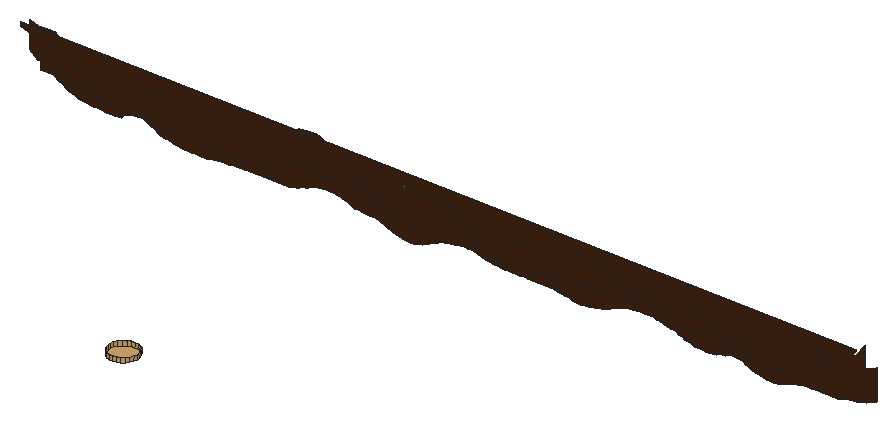
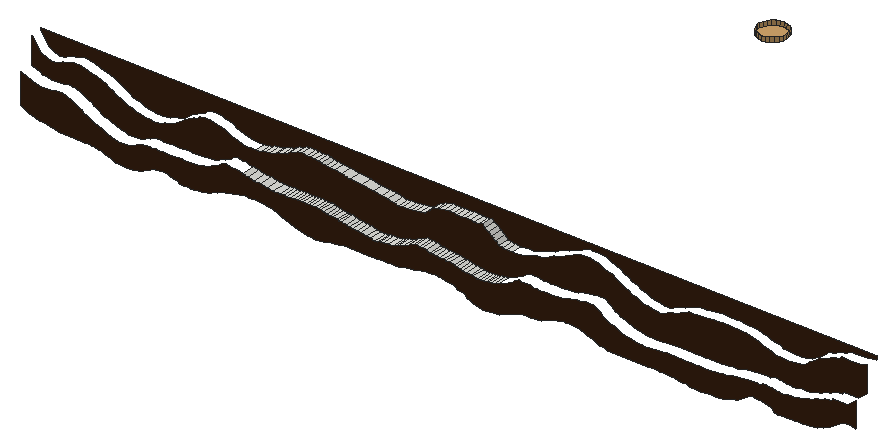
# SketchUp Ruby script. Lengths in inches.
U = 1.inch
M = Sketchup.active_model
def pt(a) = Geom::Point3d.new(a.map { |v| v * U })
def face(e, loops, mat)
  f = e.add_face(loops[0].map { |a| pt(a) })
  loops[1..].each { |l| e.add_face(l.map { |a| pt(a) }).erase! }
  f.material = f.back_material = mat if mat
  f
end
# faces: each face lists its corners as indices into pts; further lists are holes
def faces(e, pts, list, mat = nil) = list.each { |f| face(e, (f[0].is_a?(Array) ? f : [f]).map { |l| l.map { |i| pts[i] } }, mat) }
# xy, xz, yz: faces in a plane at the given z, y or x. An outline is a flat list of corners, or four numbers for a rectangle; further outlines are holes
def ring(l) = l.size == 4 ? [[l[0], l[1]], [l[2], l[1]], [l[2], l[3]], [l[0], l[3]]] : l.each_slice(2).to_a
def flat(e, list, mat, &to3) = list.each { |f| face(e, (f[0].is_a?(Array) ? f : [f]).map { |l| ring(l).map { |u, v| to3.(u, v) } }, mat) }
def xy(e, z, list, mat = nil) = flat(e, list, mat) { |x, y| [x, y, z] }
def xz(e, y, list, mat = nil) = flat(e, list, mat) { |x, z| [x, y, z] }
def yz(e, x, list, mat = nil) = flat(e, list, mat) { |y, z| [x, y, z] }
def lines(e, pts, list) = list.each { |a, b| e.add_line(pt(pts[a]), pt(pts[b])) }
# prism: a flat outline (further loops are holes) pulled along v
def prism(e, loops, v, mat = nil)
  f = face(e, loops, mat); d = Geom::Vector3d.new(v.map { |x| x * U })
  f.pushpull(f.normal.samedirection?(d) ? d.length : -d.length)
end
def box(e, o, s, mat = nil) = prism(e, [[o, [o[0] + s[0], o[1], o[2]], [o[0] + s[0], o[1] + s[1], o[2]], [o[0], o[1] + s[1], o[2]]]], [0, 0, s[2]], mat)
def at(x, y, z, deg = 0) = Geom::Transformation.translation(pt([x, y, z])) * Geom::Transformation.rotation(ORIGIN, Z_AXIS, deg.degrees)
def axes(o, x, y, z) = Geom::Transformation.new([*x, 0, *y, 0, *z, 0, *pt(o).to_a, 1])
def part(name) = M.definitions.add(name)
# library, detail: a bought-in or finely detailed component or shape, given as its bounding box
def library(name, o, s) = part(name).tap { |d| box(d.entities, o, s) }
def detail(e, o, s) = box(e.add_group.entities, o, s)
def put(e, d, t, mat = nil) = e.add_instance(d, t).tap { |i| i.material = mat if mat }
def group(e, t, mat = nil) = e.add_group.tap { |g| g.transformation = t; g.material = mat if mat }.entities
root = M.entities
M.materials.add("[Field Square Tile]").color = [211, 167, 108]
M.materials.add("[Wood Veneer 01]").color = [66, 38, 20]
xy(root,243.05,[[358.29,2398.8,358.97,2401.37]])
xy(root,243.07,[[356.4375,2398.8,357.02,2401.37]])
xy(root,243.09,[[353.125,2398.8,353.65,2401.37],[353.65,2398.8,354.17,2401.37],[354.17,2398.8,354.83,2401.37],[354.83,2398.8,355.28,2401.37]])
xy(root,249.21,[[325.92,2396.68,326.81,2398.8]])
xy(root,249.22,[[327.53,2396.68,328.4375,2398.8]])
xy(root,249.23,[[329.08,2396.68,329.98,2398.8]])
xy(root,250.6875,[[324.47,2328.39,323.81,2328.48,323.19,2328.74,322.66,2329.14,322.25,2329.68,322,2330.29,321.91,2330.96,322,2331.62,322.25,2332.24,322.66,2332.77,323.19,2333.18,323.81,2333.43,324.47,2333.52,325.13,2333.43,325.75,2333.18,326.28,2332.77,326.69,2332.24,326.95,2331.62,327.03,2330.96,326.95,2330.29,326.69,2329.68,326.28,2329.14,325.75,2328.74,325.13,2328.48]],"[Field Square Tile]")
xz(root,2396.68,[[384.34,244.87,385.25,245.01,386.1875,245.12,386.95,245.25,387.71,245.41,388.34,245.78,389.14,245.88,389.85,246.16,390.45,246.57,391.24,246.9,391.84,247.35,392.51,247.62,393.1,248.06,393.86,248.32,394.97,248.66,395.75,248.79,396.61,249.19,397.28,249.32,398.21,249.41,399.06,249.48,399.81,249.21,400.45,248.96,401.15,248.9,401.95,248.42,402.66,248.3,403.37,248.22,404.1875,248.56,405.12,249.02,406.85,251.16,406.85,251.5,252.84,251.5,252.84,250.88,254.43,250.53,256.05,250.54,257.51,250.55,258.04,250.15,258.65,249.97,259.45,249.8,260.12,249.41,260.79,249.2,261.56,249.01,262.05,248.51,262.68,248.07,263.33,247.72,263.97,247.25,264.52,246.88,265.24,246.73,265.9,246.62,266.64,246.54,267.42,246.51,268.2,246.58,269,246.59,269.8,246.69,270.51,247.03,271.2,247.2,272.17,247.39,272.8,247.78,273.58,247.89,274.58,248.18,275.22,248.29,276.11,248.35,276.84,248.4,277.83,248.4375,278.49,248.46,279.38,248.47,280.12,248.48,281.01,248.49,281.74,248.39,283.14,248.28,284.17,248.15,284.99,248.11,285.79,248.08,286.63,247.66,287.26,247.46,287.94,247.08,288.625,246.94,289.48,246.66,290.09,246.35,290.86,246.05,291.76,246.13,292.47,246.29,293.27,246.41,294.18,246.55,294.91,246.92,295.52,247.12,296.2,247.31,296.77,247.71,297.7,248.03,298.41,248.46,299.19,248.82,299.91,249.37,300.7,249.5625,301.6,249.9,302.52,250.35,303.18,250.49,303.99,250.6,305.01,250.58,305.65,250.61,306.27,250.32,306.96,250.0625,307.62,249.68,308.38,249.46,309.27,248.95,310.49,248.69,311.4,248.26,312,247.9,313.13,247.66,313.71,247.53,314.39,247.25,315.2,246.95,315.89,246.75,316.68,246.66,317.39,246.59,318.28,246.55,319.21,246.63,319.95,246.74,320.68,246.87,321.29,247.42,321.96,247.96,322.53,248.44,323.27,248.85,323.74,249.34,324.47,249.125,325.24,249.17,325.92,249.21,326.81,249.21,327.53,249.22,328.4375,249.22,329.08,249.23,329.98,249.23,330.72,249.24,331.52,249.14,332.15,248.82,332.94,248.54,333.64,248.04,334.33,247.48,335.22,247.29,336.04,247.15,336.77,247.05,337.49,247,338.4,246.96,339.125,246.94,340.04,247.04,341.1,247.36,342.28,247.43,343.93,247.6,345.91,247.98,348.11,248.1875,349.72,248.49,350.97,248.62,351.91,248.69,352.59,248.75,353.25,249.09,353.95,249.18,354.73,249.13,355.43,249.17,356.13,249.18,357.03,249.29,357.76,249.21,358.37,248.8,359.0625,248.73,359.84,248.26,360.54,248.02,361.34,247.8125,362.05,247.4,362.96,247.27,363.7,247.18,364.625,246.91,365.49,246.84,366.44,246.79,367.22,246.75,367.97,246.83,369.01,247.25,369.88,247.55,370.55,247.66,371.18,248.16,371.97,248.41,372.67,248.52,373.37,248.72,374.07,248.8,374.96,248.85,375.79,248.6875,376.33,248.26,377.02,248.06,377.91,247.55,378.62,247.19,379.43,246.63,380.0625,246.13,380.65,245.83,381.33,245.67,382.2,245.46,382.91,245.0625,383.625,244.95]],"[Wood Veneer 01]")
xz(root,2398.8,[[388.34,241.09,388.91,241.14,389.55,241.35,390.14,241.46,391.08,241.85,392.08,242.23,392.64,242.42,393.36,242.61,393.875,242.91,394.25,243.14,394.79,243.52,395.27,243.71,395.6,244.02,396.04,244.21,396.63,244.57,397.1,244.76,397.72,245.125,398.22,245.32,398.7,245.41,399.25,245.48,399.74,245.59,400.27,245.55,400.88,245.35,401.37,245.31,401.92,245.27,402.48,245.24,403.04,245.22,403.6,245.34,404.23,245.42,404.8125,245.52,405.19,245.76,405.66,245.9,406.85,246.43,406.85,251.16,405.12,249.02,404.1875,248.56,403.37,248.22,402.66,248.3,401.95,248.42,401.15,248.9,400.45,248.96,399.81,249.21,399.06,249.48,398.21,249.41,397.28,249.32,396.61,249.19,395.75,248.79,394.97,248.66,393.86,248.32,393.1,248.06,392.51,247.62,391.84,247.35,391.24,246.9,390.45,246.57,389.85,246.16,389.14,245.88,388.34,245.78,387.71,245.41,386.95,245.25,386.1875,245.12,385.25,245.01,384.34,244.87,383.625,244.95,382.91,245.0625,382.2,245.46,381.33,245.67,380.65,245.83,380.0625,246.13,379.43,246.63,378.62,247.19,377.91,247.55,377.02,248.06,376.33,248.26,375.79,248.6875,374.96,248.85,374.07,248.8,373.37,248.72,372.67,248.52,371.97,248.41,371.18,248.16,370.55,247.66,369.88,247.55,369.01,247.25,367.97,246.83,367.22,246.75,366.44,246.79,365.49,246.84,364.625,246.91,363.7,247.18,362.96,247.27,362.05,247.4,361.34,247.8125,360.54,248.02,359.84,248.26,359.0625,248.73,358.37,248.8,357.76,249.21,357.03,249.29,356.13,249.18,355.43,249.17,354.73,249.13,353.95,249.18,353.25,249.09,352.59,248.75,351.91,248.69,350.97,248.62,349.72,248.49,348.11,248.1875,345.91,247.98,343.93,247.6,342.28,247.43,341.1,247.36,340.04,247.04,339.125,246.94,338.4,246.96,337.49,247,336.77,247.05,336.04,247.15,335.22,247.29,334.33,247.48,333.64,248.04,332.94,248.54,332.15,248.82,331.52,249.14,330.72,249.24,329.98,249.23,329.08,249.23,328.4375,249.22,327.53,249.22,326.81,249.21,325.92,249.21,325.24,249.17,324.47,249.125,323.74,249.34,323.27,248.85,322.53,248.44,321.96,247.96,321.29,247.42,320.68,246.87,319.95,246.74,319.21,246.63,318.28,246.55,317.39,246.59,316.68,246.66,315.89,246.75,315.2,246.95,314.39,247.25,313.71,247.53,313.13,247.66,312,247.9,311.4,248.26,310.49,248.69,309.27,248.95,308.38,249.46,307.62,249.68,306.96,250.0625,306.27,250.32,305.65,250.61,305.01,250.58,303.99,250.6,303.18,250.49,302.52,250.35,301.6,249.9,300.7,249.5625,299.91,249.37,299.19,248.82,298.41,248.46,297.7,248.03,296.77,247.71,296.2,247.31,295.52,247.12,294.91,246.92,294.18,246.55,293.27,246.41,292.47,246.29,291.76,246.13,290.86,246.05,290.09,246.35,289.48,246.66,288.625,246.94,287.94,247.08,287.26,247.46,286.63,247.66,285.79,248.08,284.99,248.11,284.17,248.15,283.14,248.28,281.74,248.39,281.01,248.49,280.12,248.48,279.38,248.47,278.49,248.46,277.83,248.4375,276.84,248.4,276.11,248.35,275.22,248.29,274.58,248.18,273.58,247.89,272.8,247.78,272.17,247.39,271.2,247.2,270.51,247.03,269.8,246.69,269,246.59,268.2,246.58,267.42,246.51,266.64,246.54,265.9,246.62,265.24,246.73,264.52,246.88,263.97,247.25,263.33,247.72,262.68,248.07,262.05,248.51,261.56,249.01,260.79,249.2,260.12,249.41,259.45,249.8,258.65,249.97,258.04,250.15,257.51,250.55,256.05,250.54,254.43,250.53,252.84,250.88,252.84,246.2,254.41,244.96,255.8,244.9375,257.05,244.92,257.27,244.61,257.83,244.54,258.59,244.41,259.26,244.11,259.78,243.95,260.44,243.79,260.96,243.48,261.6,243.3,262.1875,243.14,262.67,243.06,263.39,242.85,263.97,242.78,264.78,242.73,265.32,242.68,265.99,242.51,266.51,242.46,267.05,242.58,267.68,242.57,268.31,242.81,268.88,242.86,269.44,242.89,270.08,242.92,270.51,242.625,271.12,242.65,271.67,242.62,272.3,242.58,272.86,242.57,273.5,242.48,274.16,242.38,274.82,242.34,275.49,242.24,276.66,241.96,277.43,241.89,278.25,241.83,278.85,241.78,279.62,241.75,280.07,241.74,280.62,241.72,281.88,241.7,282.61,241.69,283.28,241.68,283.87,241.68,284.36,241.67,285.0625,241.74,285.63,241.75,287.63,241.75,288.12,241.67,288.65,241.66,289.26,241.57,289.8,241.53,290.42,241.51,290.97,241.49,291.67,241.48,292.33,241.47,292.9,241.46,293.61,241.6,294.34,241.85,295.01,241.91,295.91,242.1,296.68,242.46,297.38,242.78,298.15,242.97,298.68,243.23,299.08,243.48,299.6,243.72,299.9375,244.12,300.41,244.39,300.89,244.73,301.375,244.87,301.96,244.95,302.64,245.01,303.29,244.81,303.86,244.7,304.34,244.67,304.95,244.55,305.49,244.51,305.95,244.25,306.7,244.11,307.26,244.04,307.88,243.99,308.6,243.95,309.1,243.93,309.79,243.91,310.36,243.89,311.06,243.88,311.71,243.94,312.35,243.95,312.91,244.1,313.54,244.13,314.02,244.15,314.54,244.17,315.06,244.18,315.66,243.8,316.2,243.43,316.81,243.09,317.2,242.875,317.7,242.68,318.29,242.51,318.8,242.21,319.4,242.11,320.08,241.96,320.64,241.89,321.1,241.85,321.62,241.8125,322.13,241.79,322.71,241.78,323.38,241.91,323.85,241.93,324.52,242.09,325.29,242.2,325.79,242.24,326.4,242.42,326.95,242.47,327.7,242.71,328.34,242.78,328.82,242.82,329.51,242.85,330.21,242.87,330.76,243.02,331.38,243.05,331.93,243.29,332.61,243.35,333.16,243.39,333.76,243.42,334.53,243.14,335.1,242.9375,335.65,242.65,336.27,242.39,337.03,242.14,337.67,241.89,338.16,241.78,339.21,241.63,339.98,241.56,340.58,241.51,341.03,241.48,341.55,241.46,342.42,241.51,343.14,241.59,344.08,241.82,344.86,241.87,345.625,241.98,346.24,242.02,346.89,242.19,347.59,242.38,348.08,242.4375,348.6,242.48,349.26,242.58,349.79,242.61,350.375,242.77,350.83,242.95,351.39,243.01,351.9,243.05,352.47,243.08,353.125,243.09,355.28,243.09,355.85,243.08,356.4375,243.07,357.02,243.07,357.68,243.0625,358.29,243.05,358.97,243.05,360.24,243.1,361.41,243.17,362.55,243.4,363.8125,243.52,364.94,243.71,365.84,243.99,366.54,244.08,367.24,244.21,367.82,244.27,368.36,244.3,369.03,244.39,369.625,244.19,370,243.88,370.48,243.59,371.03,243.33,371.58,243.22,372.07,242.92,372.55,242.75,373.11,242.6,373.67,242.52,374.23,242.47,374.8125,242.43,375.39,242.4,375.97,242.39,376.55,242.37,377.13,242.36,377.72,242.35,378.88,242.33,379.46,242.33,380.18,242.32,380.65,242.3125,381.29,242.3,381.96,242.3,382.41,242.29,383.05,242.28,383.5625,242.28,384.19,242.2,384.77,241.97,385.34,241.84,385.85,241.57,386.27,241.33,386.74,241.24,387.27,241.17,387.74,241.12]],"[Wood Veneer 01]")
xz(root,2401.37,[[321.7,236.98,322.38,237.22,323.23,237.43,323.85,237.74,324.55,238.02,324.99,238.375,325.55,238.51,326.1875,238.76,326.83,239.12,327.41,239.22,328.41,239.31,329.22,239.54,329.71,239.6,330.33,239.65,330.92,239.69,331.48,239.7,332.21,239.72,332.82,239.56,333.49,239.44,334.34,239.16,334.89,239.07,335.66,238.93,336.54,238.78,337.02,238.73,337.69,238.6875,338.38,238.66,339.05,238.65,339.83,238.64,340.45,238.63,341.14,238.625,342,238.625,342.56,238.62,347.45,238.62,348.14,238.45,348.9,238.25,349.52,238.19,350.29,238.15,350.92,237.86,351.69,237.79,352.4,237.74,353.27,237.87,353.92,237.88,355.04,238.14,356.26,238.46,357.01,238.72,357.89,239.08,358.68,239.375,359.42,239.75,360.07,239.97,360.69,240.17,361.37,240.27,362.05,240.33,362.74,240.37,363.43,240.4,364.125,240.41,364.65,240.42,365.23,240.43,365.8,240.43,366.45,240.27,367.03,240.23,367.68,239.96,368.4375,239.8,369.05,239.65,369.8125,239.5,370.4375,239.18,371.12,239.01,371.64,238.67,372.21,238.56,372.87,238.48,373.4375,238.26,374.01,238.19,374.83,238.15,375.36,238.11,376.03,238.18,376.71,238.18,377.39,238.27,377.91,238.55,378.57,238.61,379.16,238.66,379.73,239.04,380.47,239.125,381.15,239.02,381.84,238.96,382.36,238.86,382.86,238.57,383.41,238.33,384.12,238,384.95,237.71,385.49,237.59,386.09,237.51,386.68,237.45,387.25,237.42,387.98,237.4,388.66,237.47,389.26,237.5625,389.95,237.84,390.63,238.08,391.32,238.33,391.85,238.51,392.42,238.6,393.08,238.74,393.66,238.8,394.23,238.83,394.97,238.86,395.73,238.875,396.27,238.88,396.95,238.89,397.63,238.89,398.39,238.9,399.78,238.9,400.41,239.15,401.18,239.28,401.98,239.42,402.7,239.49,403.25,239.53,403.9375,239.81,404.46,239.96,405.02,240.1,406.85,240.89,406.85,246.43,405.66,245.9,405.19,245.76,404.8125,245.52,404.23,245.42,403.6,245.34,403.04,245.22,402.48,245.24,401.92,245.27,401.37,245.31,400.88,245.35,400.27,245.55,399.74,245.59,399.25,245.48,398.7,245.41,398.22,245.32,397.72,245.125,397.1,244.76,396.63,244.57,396.04,244.21,395.6,244.02,395.27,243.71,394.79,243.52,394.25,243.14,393.875,242.91,393.36,242.61,392.64,242.42,392.08,242.23,391.08,241.85,390.14,241.46,389.55,241.35,388.91,241.14,388.34,241.09,387.74,241.12,387.27,241.17,386.74,241.24,386.27,241.33,385.85,241.57,385.34,241.84,384.77,241.97,384.19,242.2,383.5625,242.28,383.05,242.28,382.41,242.29,381.96,242.3,381.29,242.3,380.65,242.3125,380.18,242.32,379.46,242.33,378.88,242.33,377.72,242.35,377.13,242.36,376.55,242.37,375.97,242.39,375.39,242.4,374.8125,242.43,374.23,242.47,373.67,242.52,373.11,242.6,372.55,242.75,372.07,242.92,371.58,243.22,371.03,243.33,370.48,243.59,370,243.88,369.625,244.19,369.03,244.39,368.36,244.3,367.82,244.27,367.24,244.21,366.54,244.08,365.84,243.99,364.94,243.71,363.8125,243.52,362.55,243.4,361.41,243.17,360.24,243.1,358.97,243.05,358.29,243.05,357.68,243.0625,357.02,243.07,356.4375,243.07,355.85,243.08,355.28,243.09,353.125,243.09,352.47,243.08,351.9,243.05,351.39,243.01,350.83,242.95,350.375,242.77,349.79,242.61,349.26,242.58,348.6,242.48,348.08,242.4375,347.59,242.38,346.89,242.19,346.24,242.02,345.625,241.98,344.86,241.87,344.08,241.82,343.14,241.59,342.42,241.51,341.55,241.46,341.03,241.48,340.58,241.51,339.98,241.56,339.21,241.63,338.16,241.78,337.67,241.89,337.03,242.14,336.27,242.39,335.65,242.65,335.1,242.9375,334.53,243.14,333.76,243.42,333.16,243.39,332.61,243.35,331.93,243.29,331.38,243.05,330.76,243.02,330.21,242.87,329.51,242.85,328.82,242.82,328.34,242.78,327.7,242.71,326.95,242.47,326.4,242.42,325.79,242.24,325.29,242.2,324.52,242.09,323.85,241.93,323.38,241.91,322.71,241.78,322.13,241.79,321.62,241.8125,321.1,241.85,320.64,241.89,320.08,241.96,319.4,242.11,318.8,242.21,318.29,242.51,317.7,242.68,317.2,242.875,316.81,243.09,316.2,243.43,315.66,243.8,315.06,244.18,314.54,244.17,314.02,244.15,313.54,244.13,312.91,244.1,312.35,243.95,311.71,243.94,311.06,243.88,310.36,243.89,309.79,243.91,309.1,243.93,308.6,243.95,307.88,243.99,307.26,244.04,306.7,244.11,305.95,244.25,305.49,244.51,304.95,244.55,304.34,244.67,303.86,244.7,303.29,244.81,302.64,245.01,301.96,244.95,301.375,244.87,300.89,244.73,300.41,244.39,299.9375,244.12,299.6,243.72,299.08,243.48,298.68,243.23,298.15,242.97,297.38,242.78,296.68,242.46,295.91,242.1,295.01,241.91,294.34,241.85,293.61,241.6,292.9,241.46,292.33,241.47,291.67,241.48,290.97,241.49,290.42,241.51,289.8,241.53,289.26,241.57,288.65,241.66,288.12,241.67,287.63,241.75,285.63,241.75,285.0625,241.74,284.36,241.67,283.87,241.68,283.28,241.68,282.61,241.69,281.88,241.7,280.62,241.72,280.07,241.74,279.62,241.75,278.85,241.78,278.25,241.83,277.43,241.89,276.66,241.96,275.49,242.24,274.82,242.34,274.16,242.38,273.5,242.48,272.86,242.57,272.3,242.58,271.67,242.62,271.12,242.65,270.51,242.625,270.08,242.92,269.44,242.89,268.88,242.86,268.31,242.81,267.68,242.57,267.05,242.58,266.51,242.46,265.99,242.51,265.32,242.68,264.78,242.73,263.97,242.78,263.39,242.85,262.67,243.06,262.1875,243.14,261.6,243.3,260.96,243.48,260.44,243.79,259.78,243.95,259.26,244.11,258.59,244.41,257.83,244.54,257.27,244.61,257.05,244.92,255.8,244.9375,254.41,244.96,252.84,246.2,252.84,241.52,254.05,241.69,255.32,241.55,256.34,240.85,256.88,240.59,257.48,240.2,258.27,239.86,258.72,239.64,259.28,239.52,259.79,239.19,260.57,239.09,261.26,239.03,261.94,238.97,262.64,238.94,263.34,238.93,264.03,238.92,265.07,238.82,265.58,238.8,266.45,238.79,267.19,238.77,267.72,238.9375,268.28,239.55,268.86,239.69,269.41,239.88,270.14,239.99,270.73,240.05,271.39,240.09,272.08,240.11,272.78,239.71,273.24,239.38,273.82,239.11,274.4,238.74,275.05,238.43,275.96,238.31,276.43,238.21,277.37,237.9,278.03,237.82,278.72,237.76,279.43,237.71,280.04,237.68,280.64,237.67,281.39,237.66,282.08,237.65,283.39,237.65,284.06,237.89,284.82,237.94,285.4375,237.98,286.29,238.1,286.84,238.13,287.6,238.15,288.23,238.26,288.98,238.28,289.61,238.3,290.46,238.32,291.18,238.33,292.41,238.33,293.09,238.34,298.66,238.34,299.17,238.59,299.99,238.72,300.68,238.86,301.19,239.18,301.78,239.35,302.34,239.52,302.89,239.85,303.53,240.03,304.1875,240.12,304.86,240.19,305.625,240.23,306.33,240.25,306.95,240.27,307.73,240.11,308.36,239.92,309.05,239.7,309.58,239.53,310.16,239.29,310.82,239.04,311.4,238.94,311.97,238.875,312.72,238.83,313.48,238.8,314.02,238.79,314.69,238.78,315.47,238.43,316.25,238.28,316.8125,237.96,317.75,237.68,318.42,237.33,318.95,237.2,319.64,237.11,320.4,237.04,321.09,237.01]],"[Wood Veneer 01]")
p = [[339.98,2398.8,241.56],[339.98,2401.37,241.56],[340.58,2401.37,241.51],[340.58,2398.8,241.51],[341.03,2401.37,241.48],[341.03,2398.8,241.48],
  [341.55,2401.37,241.46],[341.55,2398.8,241.46],[342.42,2401.37,241.51],[342.42,2398.8,241.51],[343.14,2401.37,241.59],[343.14,2398.8,241.59],
  [338.16,2398.8,241.78],[338.16,2401.37,241.78],[339.21,2401.37,241.63],[339.21,2398.8,241.63],[344.08,2401.37,241.82],[344.08,2398.8,241.82],
  [320.64,2398.8,241.89],[320.64,2401.37,241.89],[321.1,2401.37,241.85],[321.1,2398.8,241.85],[321.62,2401.37,241.8125],[321.62,2398.8,241.8125],
  [322.13,2401.37,241.79],[322.13,2398.8,241.79],[322.71,2401.37,241.78],[322.71,2398.8,241.78],[323.38,2401.37,241.91],[323.38,2398.8,241.91],
  [337.67,2398.8,241.89],[337.67,2401.37,241.89],[344.86,2401.37,241.87],[344.86,2398.8,241.87],[320.08,2398.8,241.96],[320.08,2401.37,241.96],
  [323.85,2401.37,241.93],[323.85,2398.8,241.93],[324.52,2401.37,242.09],[324.52,2398.8,242.09],[337.03,2398.8,242.14],[337.03,2401.37,242.14],
  [345.625,2401.37,241.98],[345.625,2398.8,241.98],[319.4,2398.8,242.11],[319.4,2401.37,242.11],[346.24,2401.37,242.02],[346.24,2398.8,242.02],
  [346.89,2401.37,242.19],[346.89,2398.8,242.19],[318.8,2398.8,242.21],[318.8,2401.37,242.21],[325.29,2401.37,242.2],[325.29,2398.8,242.2],
  [336.27,2398.8,242.39],[336.27,2401.37,242.39],[325.79,2401.37,242.24],[325.79,2398.8,242.24],[326.4,2401.37,242.42],[326.4,2398.8,242.42],
  [347.59,2401.37,242.38],[347.59,2398.8,242.38],[326.95,2401.37,242.47],[326.95,2398.8,242.47],[335.65,2398.8,242.65],[335.65,2401.37,242.65],
  [348.08,2401.37,242.4375],[348.08,2398.8,242.4375],[348.6,2401.37,242.48],[348.6,2398.8,242.48],[327.7,2401.37,242.71],[327.7,2398.8,242.71],
  [349.26,2401.37,242.58],[349.26,2398.8,242.58],[335.1,2398.8,242.9375],[335.1,2401.37,242.9375],[349.79,2401.37,242.61],[349.79,2398.8,242.61],
  [350.375,2401.37,242.77],[350.375,2398.8,242.77],[328.34,2401.37,242.78],[328.34,2398.8,242.78],[328.82,2401.37,242.82],[328.82,2398.8,242.82],
  [329.51,2401.37,242.85],[329.51,2398.8,242.85],[350.83,2401.37,242.95],[350.83,2398.8,242.95],[330.21,2401.37,242.87],[330.21,2398.8,242.87],
  [330.76,2401.37,243.02],[330.76,2398.8,243.02],[334.53,2398.8,243.14],[334.53,2401.37,243.14],[331.38,2401.37,243.05],[331.38,2398.8,243.05],
  [351.39,2401.37,243.01],[351.39,2398.8,243.01],[351.9,2401.37,243.05],[351.9,2398.8,243.05],[352.47,2401.37,243.08],[352.47,2398.8,243.08],
  [358.97,2398.8,243.05],[358.97,2401.37,243.05],[360.24,2401.37,243.1],[360.24,2398.8,243.1],[331.93,2401.37,243.29],[331.93,2398.8,243.29],
  [333.76,2398.8,243.42],[333.76,2401.37,243.42],[353.125,2401.37,243.09],[353.125,2398.8,243.09],[355.28,2398.8,243.09],[355.28,2401.37,243.09],
  [355.85,2401.37,243.08],[355.85,2398.8,243.08],[356.4375,2401.37,243.07],[356.4375,2398.8,243.07],[357.02,2398.8,243.07],[357.02,2401.37,243.07],
  [357.68,2401.37,243.0625],[357.68,2398.8,243.0625],[358.29,2401.37,243.05],[358.29,2398.8,243.05],[361.41,2401.37,243.17],[361.41,2398.8,243.17],
  [362.55,2401.37,243.4],[362.55,2398.8,243.4],[332.61,2401.37,243.35],[332.61,2398.8,243.35],[333.16,2401.37,243.39],[333.16,2398.8,243.39],
  [363.8125,2401.37,243.52],[363.8125,2398.8,243.52],[364.94,2401.37,243.71],[364.94,2398.8,243.71],[365.84,2401.37,243.99],[365.84,2398.8,243.99],
  [318.28,2396.68,246.55],[318.28,2398.8,246.55],[319.21,2398.8,246.63],[319.21,2396.68,246.63],[319.95,2398.8,246.74],[319.95,2396.68,246.74],
  [320.68,2398.8,246.87],[320.68,2396.68,246.87],[364.625,2396.68,246.91],[364.625,2398.8,246.91],[365.49,2398.8,246.84],[365.49,2396.68,246.84],
  [321.29,2398.8,247.42],[321.29,2396.68,247.42],[338.4,2396.68,246.96],[338.4,2398.8,246.96],[339.125,2398.8,246.94],[339.125,2396.68,246.94],
  [340.04,2398.8,247.04],[340.04,2396.68,247.04],[363.7,2396.68,247.18],[363.7,2398.8,247.18],[336.04,2396.68,247.15],[336.04,2398.8,247.15],
  [336.77,2398.8,247.05],[336.77,2396.68,247.05],[337.49,2398.8,247],[337.49,2396.68,247],[341.1,2398.8,247.36],[341.1,2396.68,247.36],
  [335.22,2396.68,247.29],[335.22,2398.8,247.29],[362.96,2396.68,247.27],[362.96,2398.8,247.27],[334.33,2396.68,247.48],[334.33,2398.8,247.48],
  [362.05,2396.68,247.4],[362.05,2398.8,247.4],[321.96,2398.8,247.96],[321.96,2396.68,247.96],[342.28,2398.8,247.43],[342.28,2396.68,247.43],
  [343.93,2398.8,247.6],[343.93,2396.68,247.6],[361.34,2396.68,247.8125],[361.34,2398.8,247.8125],[333.64,2396.68,248.04],[333.64,2398.8,248.04],
  [345.91,2398.8,247.98],[345.91,2396.68,247.98],[360.54,2396.68,248.02],[360.54,2398.8,248.02],[322.53,2398.8,248.44],[322.53,2396.68,248.44],
  [332.94,2396.68,248.54],[332.94,2398.8,248.54],[348.11,2398.8,248.1875],[348.11,2396.68,248.1875],[359.84,2396.68,248.26],[359.84,2398.8,248.26],
  [349.72,2398.8,248.49],[349.72,2396.68,248.49],[359.0625,2396.68,248.73],[359.0625,2398.8,248.73],[323.27,2398.8,248.85],[323.27,2396.68,248.85],
  [332.15,2396.68,248.82],[332.15,2398.8,248.82],[350.97,2398.8,248.62],[350.97,2396.68,248.62],[351.91,2398.8,248.69],[351.91,2396.68,248.69],
  [352.59,2398.8,248.75],[352.59,2396.68,248.75],[358.37,2396.68,248.8],[358.37,2398.8,248.8],[331.52,2396.68,249.14],[331.52,2398.8,249.14],
  [353.25,2398.8,249.09],[353.25,2396.68,249.09],[357.76,2396.68,249.21],[357.76,2398.8,249.21],[323.74,2398.8,249.34],[323.74,2396.68,249.34],
  [324.47,2398.8,249.125],[324.47,2396.68,249.125],[325.24,2398.8,249.17],[325.24,2396.68,249.17],[330.72,2396.68,249.24],[330.72,2398.8,249.24],
  [353.95,2398.8,249.18],[353.95,2396.68,249.18],[354.73,2398.8,249.13],[354.73,2396.68,249.13],[355.43,2398.8,249.17],[355.43,2396.68,249.17],
  [325.92,2398.8,249.21],[325.92,2396.68,249.21],[326.81,2396.68,249.21],[326.81,2398.8,249.21],[327.53,2398.8,249.22],[327.53,2396.68,249.22],
  [328.4375,2396.68,249.22],[328.4375,2398.8,249.22],[329.08,2398.8,249.23],[329.08,2396.68,249.23],[329.98,2396.68,249.23],[329.98,2398.8,249.23],
  [356.13,2398.8,249.18],[356.13,2396.68,249.18],[357.03,2398.8,249.29],[357.03,2396.68,249.29],[324.47,2328.39,251.5],[323.81,2328.48,251.5],
  [323.81,2328.48,250.6875],[324.47,2328.39,250.6875],[325.13,2328.48,251.5],[325.13,2328.48,250.6875],[323.19,2328.74,251.5],[323.19,2328.74,250.6875],
  [325.75,2328.74,251.5],[325.75,2328.74,250.6875],[322.66,2329.14,251.5],[322.66,2329.14,250.6875],[326.28,2329.14,251.5],[326.28,2329.14,250.6875],
  [322.25,2329.68,251.5],[322.25,2329.68,250.6875],[326.69,2329.68,251.5],[326.69,2329.68,250.6875],[322,2330.29,251.5],[322,2330.29,250.6875],
  [326.95,2330.29,251.5],[326.95,2330.29,250.6875],[321.91,2330.96,251.5],[321.91,2330.96,250.6875],[327.03,2330.96,251.5],[327.03,2330.96,250.6875],
  [322,2331.62,251.5],[322,2331.62,250.6875],[326.95,2331.62,251.5],[326.95,2331.62,250.6875],[322.25,2332.24,251.5],[322.25,2332.24,250.6875],
  [326.69,2332.24,251.5],[326.69,2332.24,250.6875],[322.66,2332.77,251.5],[322.66,2332.77,250.6875],[326.28,2332.77,251.5],[326.28,2332.77,250.6875],
  [323.19,2333.18,251.5],[323.19,2333.18,250.6875],[325.75,2333.18,251.5],[325.75,2333.18,250.6875],[323.81,2333.43,251.5],[323.81,2333.43,250.6875],
  [325.13,2333.43,251.5],[325.13,2333.43,250.6875],[324.47,2333.52,251.5],[324.47,2333.52,250.6875]]
faces(root,p,[[0,1,2,3],[3,2,4,5],[5,4,6,7],[7,6,8,9],[9,8,10,11],[12,13,14,15],[15,14,1,0],[11,10,16,17],
  [18,19,20,21],[21,20,22,23],[23,22,24,25],[25,24,26,27],[27,26,28,29],[30,31,13,12],[17,16,32,33],[34,35,19,18],
  [29,28,36,37],[37,36,38,39],[40,41,31,30],[33,32,42,43],[44,45,35,34],[43,42,46,47],[47,46,48,49],[50,51,45,44],
  [39,38,52,53],[54,55,41,40],[53,52,56,57],[57,56,58,59],[49,48,60,61],[59,58,62,63],[64,65,55,54],[61,60,66,67],
  [67,66,68,69],[63,62,70,71],[69,68,72,73],[74,75,65,64],[73,72,76,77],[77,76,78,79],[71,70,80,81],[81,80,82,83],
  [83,82,84,85],[79,78,86,87],[85,84,88,89],[89,88,90,91],[92,93,75,74],[91,90,94,95],[87,86,96,97],[97,96,98,99],
  [99,98,100,101],[102,103,104,105],[95,94,106,107],[108,109,93,92],[101,100,110,111],[112,113,114,115],[115,114,116,117],[118,119,120,121],
  [121,120,122,123],[105,104,124,125],[125,124,126,127],[107,106,128,129],[129,128,130,131],[131,130,109,108],[127,126,132,133],[133,132,134,135],
  [135,134,136,137],[138,139,140,141],[141,140,142,143],[143,142,144,145],[146,147,148,149],[145,144,150,151],[152,153,154,155],[155,154,156,157],
  [158,159,147,146],[160,161,162,163],[163,162,164,165],[165,164,153,152],[157,156,166,167],[168,169,161,160],[170,171,159,158],[172,173,169,168],
  [174,175,171,170],[151,150,176,177],[167,166,178,179],[179,178,180,181],[182,183,175,174],[184,185,173,172],[181,180,186,187],[188,189,183,182],
  [177,176,190,191],[192,193,185,184],[187,186,194,195],[196,197,189,188],[195,194,198,199],[200,201,197,196],[191,190,202,203],[204,205,193,192],
  [199,198,206,207],[207,206,208,209],[209,208,210,211],[212,213,201,200],[214,215,205,204],[211,210,216,217],[218,219,213,212],[203,202,220,221],
  [221,220,222,223],[223,222,224,225],[226,227,215,214],[217,216,228,229],[229,228,230,231],[231,230,232,233],[225,224,234,235],[236,237,238,239],
  [240,241,242,243],[244,245,227,226],[233,232,246,247],[247,246,248,249],[249,248,219,218]])
faces(root,p,[[250,251,252,253],[254,250,253,255],[251,256,257,252],[258,254,255,259],[256,260,261,257],[262,258,259,263],[260,264,265,261],[266,262,263,267],
  [264,268,269,265],[270,266,267,271],[268,272,273,269],[274,270,271,275],[272,276,277,273],[278,274,275,279],[276,280,281,277],[282,278,279,283],
  [280,284,285,281],[286,282,283,287],[284,288,289,285],[290,286,287,291],[288,292,293,289],[294,290,291,295],[292,296,297,293],[296,294,295,297]],"[Field Square Tile]")
